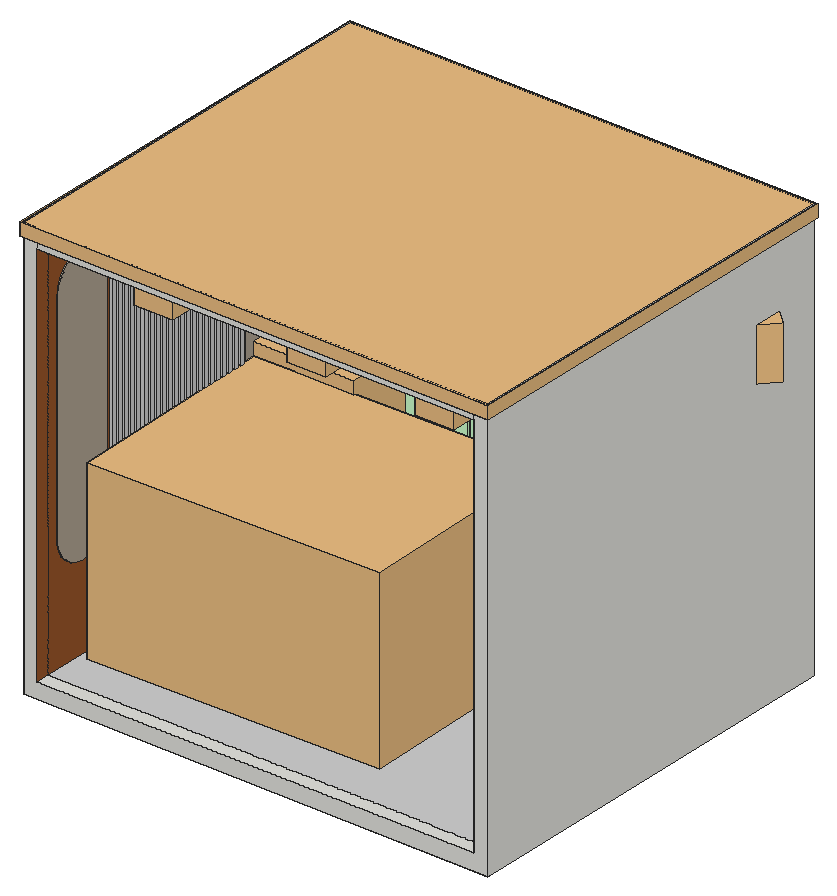
# SketchUp Ruby script. Lengths in inches.
U = 1.inch
M = Sketchup.active_model
def pt(a) = Geom::Point3d.new(a.map { |v| v * U })
def face(e, loops, mat)
  f = e.add_face(loops[0].map { |a| pt(a) })
  loops[1..].each { |l| e.add_face(l.map { |a| pt(a) }).erase! }
  f.material = f.back_material = mat if mat
  f
end
# faces: each face lists its corners as indices into pts; further lists are holes
def faces(e, pts, list, mat = nil) = list.each { |f| face(e, (f[0].is_a?(Array) ? f : [f]).map { |l| l.map { |i| pts[i] } }, mat) }
# xy, xz, yz: faces in a plane at the given z, y or x. An outline is a flat list of corners, or four numbers for a rectangle; further outlines are holes
def ring(l) = l.size == 4 ? [[l[0], l[1]], [l[2], l[1]], [l[2], l[3]], [l[0], l[3]]] : l.each_slice(2).to_a
def flat(e, list, mat, &to3) = list.each { |f| face(e, (f[0].is_a?(Array) ? f : [f]).map { |l| ring(l).map { |u, v| to3.(u, v) } }, mat) }
def xy(e, z, list, mat = nil) = flat(e, list, mat) { |x, y| [x, y, z] }
def xz(e, y, list, mat = nil) = flat(e, list, mat) { |x, z| [x, y, z] }
def yz(e, x, list, mat = nil) = flat(e, list, mat) { |y, z| [x, y, z] }
def lines(e, pts, list) = list.each { |a, b| e.add_line(pt(pts[a]), pt(pts[b])) }
# prism: a flat outline (further loops are holes) pulled along v
def prism(e, loops, v, mat = nil)
  f = face(e, loops, mat); d = Geom::Vector3d.new(v.map { |x| x * U })
  f.pushpull(f.normal.samedirection?(d) ? d.length : -d.length)
end
def box(e, o, s, mat = nil) = prism(e, [[o, [o[0] + s[0], o[1], o[2]], [o[0] + s[0], o[1] + s[1], o[2]], [o[0], o[1] + s[1], o[2]]]], [0, 0, s[2]], mat)
def at(x, y, z, deg = 0) = Geom::Transformation.translation(pt([x, y, z])) * Geom::Transformation.rotation(ORIGIN, Z_AXIS, deg.degrees)
def axes(o, x, y, z) = Geom::Transformation.new([*x, 0, *y, 0, *z, 0, *pt(o).to_a, 1])
def part(name) = M.definitions.add(name)
# library, detail: a bought-in or finely detailed component or shape, given as its bounding box
def library(name, o, s) = part(name).tap { |d| box(d.entities, o, s) }
def detail(e, o, s) = box(e.add_group.entities, o, s)
def put(e, d, t, mat = nil) = e.add_instance(d, t).tap { |i| i.material = mat if mat }
def group(e, t, mat = nil) = e.add_group.tap { |g| g.transformation = t; g.material = mat if mat }.entities
root = M.entities
M.materials.add("[0007_MistyRose]").color = [175, 163, 145]
M.materials.add("[0032_Moccasin]").color = [255, 228, 181]
M.materials.add("[0035_Tan]").color = [210, 180, 140]
M.materials.add("[0067_PaleGreen]").color = [152, 251, 152]
M.materials.add("[Carrera Marble]").color = [207, 207, 207]
M.materials.add("[Color C01]").color = [255, 229, 204]
M.materials.add("[Color G01]").color = [204, 255, 204]
M.materials.add("[Color M04]").color = [142, 142, 142]
M.materials.add("[Mirror 02]").color = [229, 229, 229]
M.materials.add("[Wood Cherry Original]").color = [152, 86, 42]
c1 = library("Spot Light",[-5.1,-5.1,-11.05],[10.2,10.2,11.05])
c2 = library("Spot Light\#1",[-5.1,-5.1,-11.05],[10.2,10.2,11.05])
c3 = library("Spot Light\#2",[-5.1,-5.1,-11.05],[10.2,10.2,11.05])
c4 = library("Spot Light\#3",[-5.1,-5.1,-11.05],[10.2,10.2,11.05])
c5 = library("Spot Light\#4",[-5.1,-5.1,-11.05],[10.2,10.2,11.05])
c6 = library("Spot Light\#5",[-5.1,-5.1,-11.05],[10.2,10.2,11.05])
c7 = library("Spot Light\#7",[-5.1,-5.1,-11.05],[10.2,10.2,11.05])
c8 = library("Tyler Platform Bed",[-34.22,-45.98,0],[68.44,91.98,40.05])
c9 = library("False Aralia 002",[-20.33,-19.19,0],[40.48,38.23,49.87])
c10 = library("Books 297 001 004",[-3.55,-2.96,-0.03],[7.44,5.56,6.72])
c11 = library("Toy 155 013",[-1.73,-1.4375,0],[3.14,2.99,4.15])
c12 = library("Candle 003",[-2.76,-2.76,0],[5.52,5.52,9.79])
c13 = library("Peperomia 450 001",[-6.6875,-10.1875,-9.42],[16.7,12.74,19.03])
c14 = library("Door 243 059",[-21.8,-2.74,0],[43.6,5.48,83.78])
c15 = library("Television screen",[0,1.41,1.14],[35.92,0.28,20.21])
c16 = library("Dome Light",[-12,-12,0],[24,24,12])
c17 = library("Group\#2",[-0.5,-0.5,0],[122.125,107.5,3.25])
c18 = library("Group\#3",[-0.5,-0.5,0],[93.47,84.17,1.0625])
c19 = library("Group\#4",[-0.5,-0.5,0],[1.8125,34.77,40.81])
c20 = library("Group\#5",[-0.5,-0.5,0],[1.8125,35.32,39.97])
c21 = library("Group\#6",[-0.5,-0.5,0],[1.8125,69.04,80.78])
xy(root,0,[[0,0,121.125,106.5]])
xy(root,4.25,[[3.58,0,117.55,3.58]])
xy(root,4.25,[[3.58,3.58,115.3,3.58,115.3,102.92,111.55,102.92,111.55,106.5,74.8,106.5,74.8,102.92,70.3,102.92,70.3,88.61,3.58,88.61]],"[Carrera Marble]")
xy(root,6.57,[[4.27,86.61,46.77,88.61],[46.96,86.92,69.48,88.61]],"[0067_PaleGreen]")
xy(root,8.19,[[48.58,86.92,67.86,87.48]],"[0067_PaleGreen]")
xy(root,13.1875,[[115.3,87.05,120.8,100.98]],"[Color M04]")
xy(root,20.98,[[115.3,87.05,120.8,100.98]],"[Color M04]")
xy(root,21.98,[[115.3,87.05,120.8,100.98]],"[Color M04]")
xy(root,26.6875,[[3.58,47.13,4.8125,48.23],[3.58,49.22,4.8125,50.2],[3.58,51.19,4.8125,52.17],[3.58,53.16,4.8125,54.14],[3.58,55.13,4.8125,56.11],
  [3.58,57.17,4.8125,58.08],[3.58,59.07,4.8125,60.05],[3.58,61.04,4.8125,62.02],[3.58,63.01,4.8125,63.99],[3.58,64.8,4.8125,65.96]])
xy(root,26.6875,[[3.58,23.42,4.52,24.59],[3.58,25.58,4.52,26.56],[3.58,27.55,4.52,28.53],[3.58,29.52,4.52,30.5],[3.58,31.49,4.52,32.47],
  [3.58,33.46,4.8125,34.4375],[3.58,35.43,4.8125,36.41],[3.58,37.4,4.8125,38.38],[3.58,39.37,4.8125,40.35],[3.58,41.28,4.8125,42.32],
  [3.58,43.3125,4.8125,44.29],[3.58,45.28,4.8125,46.26]],"[Carrera Marble]")
xy(root,29.77,[[115.3,87.05,120.8,100.98]],"[Color M04]")
xy(root,30.77,[[115.3,87.05,120.8,100.98]],"[Color M04]")
xy(root,38.5625,[[115.3,87.05,120.8,100.98]],"[Color M04]")
xy(root,39.5625,[[115.3,87.05,120.8,100.98]],"[Color M04]")
xy(root,47.35,[[115.3,87.05,120.8,100.98]],"[Color M04]")
xy(root,48.35,[[115.3,87.05,120.8,100.98]],"[Color M04]")
xy(root,56.15,[[115.3,87.05,120.8,100.98]],"[Color M04]")
xy(root,57.15,[[115.3,87.05,120.8,100.98]],"[Color M04]")
xy(root,64.9375,[[115.3,87.05,120.8,100.98]],"[Color M04]")
xy(root,65.9375,[[115.3,87.05,120.8,100.98]],"[Color M04]")
xy(root,73.73,[[115.3,87.05,120.8,100.98]],"[Color M04]")
xy(root,74.73,[[115.3,87.05,120.8,100.98]],"[Color M04]")
xy(root,82.52,[[115.3,87.05,120.8,100.98]],"[Color M04]")
xy(root,83.52,[[115.3,87.05,120.8,100.98]],"[Color M04]")
xy(root,88.1875,[[74.8,102.92,111.55,106.5]])
xy(root,90.58,[[48.58,86.92,67.86,87.48]],"[0067_PaleGreen]")
xy(root,92.21,[[4.27,86.61,46.77,88.61],[46.96,86.92,69.48,88.61]],"[Color G01]")
xy(root,92.3125,[[116.11,14.57,116.73,82.61]])
xy(root,92.3125,[[115.3,87.05,120.8,100.98]],"[Color M04]")
xy(root,93.21,[[3.58,88.61,70.3,102.92]],"[0032_Moccasin]")
xy(root,99.8125,[[3.58,23.42,4.52,24.59],[3.58,25.58,4.52,26.56],[3.58,27.55,4.52,28.53],[3.58,29.52,4.52,30.5],[3.58,31.49,4.52,32.47],
  [3.58,33.46,4.8125,34.4375],[3.58,35.43,4.8125,36.41],[3.58,37.4,4.8125,38.38],[3.58,39.37,4.8125,40.35],[3.58,41.28,4.8125,42.32],
  [3.58,43.3125,4.8125,44.29],[3.58,45.28,4.8125,46.26],[3.58,47.13,4.8125,48.23],[3.58,49.22,4.8125,50.2],[3.58,51.19,4.8125,52.17],
  [3.58,53.16,4.8125,54.14],[3.58,55.13,4.8125,56.11],[3.58,57.17,4.8125,58.08],[3.58,59.07,4.8125,60.05],[3.58,61.04,4.8125,62.02],
  [3.58,63.01,4.8125,63.99],[3.58,64.8,4.8125,65.96]],"[Carrera Marble]")
xy(root,103.5,[[[18.2,9.625,17.55,9.67,16.91,9.8,16.29,10.01,15.7,10.3,15.16,10.66,14.67,11.09,14.24,11.58,13.875,12.125,13.58,12.71,13.375,13.33,13.25,13.97,13.2,14.625,13.2,88.3,13.25,88.95,13.375,89.59,13.58,90.21,13.875,90.8,14.24,91.34,14.67,91.83,15.16,92.26,15.7,92.625,16.29,92.92,16.91,93.125,17.55,93.25,18.2,93.3,100.67,93.3,101.32,93.25,101.96,93.125,102.58,92.92,103.17,92.625,103.71,92.26,104.21,91.83,104.64,91.34,105,90.8,105.29,90.21,105.5,89.59,105.63,88.95,105.67,88.3,105.67,14.625,105.63,13.97,105.5,13.33,105.29,12.71,105,12.125,104.64,11.58,104.21,11.09,103.71,10.66,103.17,10.3,102.58,10.01,101.96,9.8,101.32,9.67,100.67,9.625],[39.02,30.45,79.85,30.45,80.5,30.49,81.15,30.62,81.76,30.83,82.35,31.12,82.89,31.48,83.39,31.91,83.82,32.4,84.18,32.95,84.47,33.53,84.68,34.15,84.81,34.79,84.85,35.45,84.85,67.48,84.81,68.13,84.68,68.77,84.47,69.39,84.18,69.98,83.82,70.52,83.39,71.01,82.89,71.44,82.35,71.81,81.76,72.1,81.15,72.31,80.5,72.43,79.85,72.48,39.02,72.48,38.37,72.43,37.73,72.31,37.11,72.1,36.52,71.81,35.98,71.44,35.49,71.01,35.06,70.52,34.69,69.98,34.4,69.39,34.19,68.77,34.07,68.13,34.02,67.48,34.02,35.45,34.07,34.79,34.19,34.15,34.4,33.53,34.69,32.95,35.06,32.4,35.49,31.91,35.98,31.48,36.52,31.12,37.11,30.83,37.73,30.62,38.37,30.49],[22.83,78.98,23.7,79.1,24.52,79.44,25.22,79.97,25.75,80.67,26.09,81.48,26.2,82.36,26.09,83.23,25.75,84.05,25.22,84.74,24.52,85.28,23.7,85.62,22.83,85.73,21.96,85.62,21.14,85.28,20.44,84.74,19.91,84.05,19.57,83.23,19.45,82.36,19.57,81.48,19.91,80.67,20.44,79.97,21.14,79.44,21.96,79.1],[96.05,79.11,96.89,79.22,97.67,79.54,98.34,80.06,98.86,80.73,99.18,81.52,99.3,82.36,99.18,83.2,98.86,83.98,98.34,84.66,97.67,85.17,96.89,85.5,96.05,85.61,95.2,85.5,94.42,85.17,93.75,84.66,93.23,83.98,92.91,83.2,92.8,82.36,92.91,81.52,93.23,80.73,93.75,80.06,94.42,79.54,95.2,79.22],[96.05,15.87,96.84,15.97,97.58,16.28,98.21,16.76,98.7,17.4,99,18.14,99.11,18.93,99,19.72,98.7,20.46,98.21,21.1,97.58,21.58,96.84,21.89,96.05,21.99,95.25,21.89,94.51,21.58,93.88,21.1,93.39,20.46,93.09,19.72,92.98,18.93,93.09,18.14,93.39,17.4,93.88,16.76,94.51,16.28,95.25,15.97],[22.83,16.06,23.57,16.15,24.27,16.44,24.86,16.9,25.32,17.49,25.61,18.1875,25.7,18.93,25.61,19.67,25.32,20.37,24.86,20.96,24.27,21.42,23.57,21.71,22.83,21.81,22.09,21.71,21.39,21.42,20.8,20.96,20.34,20.37,20.05,19.67,19.95,18.93,20.05,18.1875,20.34,17.49,20.8,16.9,21.39,16.44,22.09,16.15],[62.49,80,63.1,80.08,63.67,80.3125,64.15,80.6875,64.53,81.18,64.76,81.75,64.85,82.36,64.76,82.97,64.53,83.54,64.15,84.03,63.67,84.4,63.1,84.64,62.49,84.72,61.875,84.64,61.3,84.4,60.82,84.03,60.44,83.54,60.21,82.97,60.125,82.36,60.21,81.75,60.44,81.18,60.82,80.6875,61.3,80.3125,61.875,80.08],[62.49,16.81,63.04,16.88,63.55,17.09,63.99,17.43,64.33,17.87,64.54,18.38,64.61,18.93,64.54,19.48,64.33,19.99,63.99,20.43,63.55,20.77,63.04,20.98,62.49,21.06,61.94,20.98,61.42,20.77,60.98,20.43,60.64,19.99,60.43,19.48,60.36,18.93,60.43,18.38,60.64,17.87,60.98,17.43,61.42,17.09,61.94,16.88]]],"[Color M04]")
xy(root,103.75,[[96.05,79.11,95.2,79.22,94.42,79.54,93.75,80.06,93.23,80.73,92.91,81.52,92.8,82.36,92.91,83.2,93.23,83.98,93.75,84.66,94.42,85.17,95.2,85.5,96.05,85.61,96.89,85.5,97.67,85.17,98.34,84.66,98.86,83.98,99.18,83.2,99.3,82.36,99.18,81.52,98.86,80.73,98.34,80.06,97.67,79.54,96.89,79.22]],"[Color M04]")
xy(root,103.8125,[[22.83,16.06,22.09,16.15,21.39,16.44,20.8,16.9,20.34,17.49,20.05,18.1875,19.95,18.93,20.05,19.67,20.34,20.37,20.8,20.96,21.39,21.42,22.09,21.71,22.83,21.81,23.57,21.71,24.27,21.42,24.86,20.96,25.32,20.37,25.61,19.67,25.7,18.93,25.61,18.1875,25.32,17.49,24.86,16.9,24.27,16.44,23.57,16.15]],"[Color M04]")
xy(root,103.875,[[22.83,78.98,21.96,79.1,21.14,79.44,20.44,79.97,19.91,80.67,19.57,81.48,19.45,82.36,19.57,83.23,19.91,84.05,20.44,84.74,21.14,85.28,21.96,85.62,22.83,85.73,23.7,85.62,24.52,85.28,25.22,84.74,25.75,84.05,26.09,83.23,26.2,82.36,26.09,81.48,25.75,80.67,25.22,79.97,24.52,79.44,23.7,79.1],[62.49,80,61.875,80.08,61.3,80.3125,60.82,80.6875,60.44,81.18,60.21,81.75,60.125,82.36,60.21,82.97,60.44,83.54,60.82,84.03,61.3,84.4,61.875,84.64,62.49,84.72,63.1,84.64,63.67,84.4,64.15,84.03,64.53,83.54,64.76,82.97,64.85,82.36,64.76,81.75,64.53,81.18,64.15,80.6875,63.67,80.3125,63.1,80.08]],"[Color M04]")
xy(root,104.0625,[[96.05,15.87,95.25,15.97,94.51,16.28,93.88,16.76,93.39,17.4,93.09,18.14,92.98,18.93,93.09,19.72,93.39,20.46,93.88,21.1,94.51,21.58,95.25,21.89,96.05,21.99,96.84,21.89,97.58,21.58,98.21,21.1,98.7,20.46,99,19.72,99.11,18.93,99,18.14,98.7,17.4,98.21,16.76,97.58,16.28,96.84,15.97],[62.49,16.81,61.94,16.88,61.42,17.09,60.98,17.43,60.64,17.87,60.43,18.38,60.36,18.93,60.43,19.48,60.64,19.99,60.98,20.43,61.42,20.77,61.94,20.98,62.49,21.06,63.04,20.98,63.55,20.77,63.99,20.43,64.33,19.99,64.54,19.48,64.61,18.93,64.54,18.38,64.33,17.87,63.99,17.43,63.55,17.09,63.04,16.88]],"[Color M04]")
xy(root,105.375,[[[3.58,0,3.58,102.92,115.3,102.92,115.3,3.58,117.55,3.58,117.55,0],[18.2,9.625,100.67,9.625,101.32,9.67,101.96,9.8,102.58,10.01,103.17,10.3,103.71,10.66,104.21,11.09,104.64,11.58,105,12.125,105.29,12.71,105.5,13.33,105.63,13.97,105.67,14.625,105.67,88.3,105.63,88.95,105.5,89.59,105.29,90.21,105,90.8,104.64,91.34,104.21,91.83,103.71,92.26,103.17,92.625,102.58,92.92,101.96,93.125,101.32,93.25,100.67,93.3,18.2,93.3,17.55,93.25,16.91,93.125,16.29,92.92,15.7,92.625,15.16,92.26,14.67,91.83,14.24,91.34,13.875,90.8,13.58,90.21,13.375,89.59,13.25,88.95,13.2,88.3,13.2,14.625,13.25,13.97,13.375,13.33,13.58,12.71,13.875,12.125,14.24,11.58,14.67,11.09,15.16,10.66,15.7,10.3,16.29,10.01,16.91,9.8,17.55,9.67]]],"[Color C01]")
xy(root,109.25,[[39.02,30.45,38.37,30.49,37.73,30.62,37.11,30.83,36.52,31.12,35.98,31.48,35.49,31.91,35.06,32.4,34.69,32.95,34.4,33.53,34.19,34.15,34.07,34.79,34.02,35.45,34.02,67.48,34.07,68.13,34.19,68.77,34.4,69.39,34.69,69.98,35.06,70.52,35.49,71.01,35.98,71.44,36.52,71.81,37.11,72.1,37.73,72.31,38.37,72.43,39.02,72.48,79.85,72.48,80.5,72.43,81.15,72.31,81.76,72.1,82.35,71.81,82.89,71.44,83.39,71.01,83.82,70.52,84.18,69.98,84.47,69.39,84.68,68.77,84.81,68.13,84.85,67.48,84.85,35.45,84.81,34.79,84.68,34.15,84.47,33.53,84.18,32.95,83.82,32.4,83.39,31.91,82.89,31.48,82.35,31.12,81.76,30.83,81.15,30.62,80.5,30.49,79.85,30.45]],"[Color M04]")
xz(root,0,[[0,0,121.125,0,121.125,110.375,117.55,110.375,117.55,4.25,3.58,4.25,3.58,110.375,0,110.375],[3.58,105.375,117.55,110.375]])
xz(root,3.58,[[115.3,4.25,117.55,105.375]],"[Color C01]")
xz(root,9.625,[[18.2,103.5,100.67,104.3125]],"[Color M04]")
xz(root,14.57,[[116.11,11.53,116.73,92.3125]])
xz(root,23.42,[[3.58,26.6875,4.52,99.8125]],"[Carrera Marble]")
xz(root,24.59,[[3.58,26.6875,4.52,99.8125]],"[Carrera Marble]")
xz(root,25.58,[[3.58,26.6875,4.52,99.8125]],"[Carrera Marble]")
xz(root,26.56,[[3.58,26.6875,4.52,99.8125]],"[Carrera Marble]")
xz(root,27.55,[[3.58,26.6875,4.52,99.8125]],"[Carrera Marble]")
xz(root,28.53,[[3.58,26.6875,4.52,99.8125]],"[Carrera Marble]")
xz(root,29.52,[[3.58,26.6875,4.52,99.8125]],"[Carrera Marble]")
xz(root,30.45,[[39.02,103.5,79.85,107.125]],"[Color M04]")
xz(root,30.5,[[3.58,26.6875,4.52,99.8125]],"[Carrera Marble]")
xz(root,31.49,[[3.58,26.6875,4.52,99.8125]],"[Carrera Marble]")
xz(root,32.47,[[3.58,26.6875,4.52,99.8125]],"[Carrera Marble]")
xz(root,33.46,[[3.58,26.6875,4.8125,99.8125]],"[Carrera Marble]")
xz(root,34.4375,[[3.58,26.6875,4.8125,99.8125]],"[Carrera Marble]")
xz(root,35.43,[[3.58,26.6875,4.8125,99.8125]],"[Carrera Marble]")
xz(root,36.41,[[3.58,26.6875,4.8125,99.8125]],"[Carrera Marble]")
xz(root,37.4,[[3.58,26.6875,4.8125,99.8125]],"[Carrera Marble]")
xz(root,38.38,[[3.58,26.6875,4.8125,99.8125]],"[Carrera Marble]")
xz(root,39.37,[[3.58,26.6875,4.8125,99.8125]],"[Carrera Marble]")
xz(root,40.35,[[3.58,26.6875,4.8125,99.8125]],"[Carrera Marble]")
xz(root,41.28,[[3.58,26.6875,4.8125,99.8125]],"[Carrera Marble]")
xz(root,42.32,[[3.58,26.6875,4.8125,99.8125]],"[Carrera Marble]")
xz(root,43.3125,[[3.58,26.6875,4.8125,99.8125]],"[Carrera Marble]")
xz(root,44.29,[[3.58,26.6875,4.8125,99.8125]],"[Carrera Marble]")
xz(root,45.28,[[3.58,26.6875,4.8125,99.8125]],"[Carrera Marble]")
xz(root,46.26,[[3.58,26.6875,4.8125,99.8125]],"[Carrera Marble]")
xz(root,47.13,[[3.58,26.6875,4.8125,99.8125]],"[Carrera Marble]")
xz(root,48.23,[[3.58,26.6875,4.8125,99.8125]],"[Carrera Marble]")
xz(root,49.22,[[3.58,26.6875,4.8125,99.8125]],"[Carrera Marble]")
xz(root,50.2,[[3.58,26.6875,4.8125,99.8125]],"[Carrera Marble]")
xz(root,51.19,[[3.58,26.6875,4.8125,99.8125]],"[Carrera Marble]")
xz(root,52.17,[[3.58,26.6875,4.8125,99.8125]],"[Carrera Marble]")
xz(root,53.16,[[3.58,26.6875,4.8125,99.8125]],"[Carrera Marble]")
xz(root,54.14,[[3.58,26.6875,4.8125,99.8125]],"[Carrera Marble]")
xz(root,55.13,[[3.58,26.6875,4.8125,99.8125]],"[Carrera Marble]")
xz(root,56.11,[[3.58,26.6875,4.8125,99.8125]],"[Carrera Marble]")
xz(root,57.17,[[3.58,26.6875,4.8125,99.8125]],"[Carrera Marble]")
xz(root,58.08,[[3.58,26.6875,4.8125,99.8125]],"[Carrera Marble]")
xz(root,59.07,[[3.58,26.6875,4.8125,99.8125]],"[Carrera Marble]")
xz(root,60.05,[[3.58,26.6875,4.8125,99.8125]],"[Carrera Marble]")
xz(root,61.04,[[3.58,26.6875,4.8125,99.8125]],"[Carrera Marble]")
xz(root,62.02,[[3.58,26.6875,4.8125,99.8125]],"[Carrera Marble]")
xz(root,63.01,[[3.58,26.6875,4.8125,99.8125]],"[Carrera Marble]")
xz(root,63.99,[[3.58,26.6875,4.8125,99.8125]],"[Carrera Marble]")
xz(root,64.8,[[3.58,26.6875,4.8125,99.8125]],"[Carrera Marble]")
xz(root,65.96,[[3.58,26.6875,4.8125,99.8125]],"[Carrera Marble]")
xz(root,72.48,[[39.02,103.5,79.85,107.125]],"[Color M04]")
xz(root,86.61,[[4.27,6.57,46.77,92.21]],"[Color G01]")
xz(root,86.61,[[58.22,21.78,60.06,22.05,61.74,22.83,63.13,24.0625,64.12,25.64,64.57,27.29,64.57,77.72,64.36,79.37,63.72,80.9,62.71,82.22,61.4,83.23,59.86,83.86,58.22,84.08,56.57,83.86,55.04,83.23,53.73,82.22,52.72,80.9,52.08,79.37,51.86,77.72,51.86,27.29,52.32,25.64,53.3,24.0625,54.7,22.83,56.38,22.05]],"[Mirror 02]")
xz(root,86.92,[[[46.96,6.57,69.48,92.21],[48.58,8.19,67.86,90.58]]],"[Color G01]")
xz(root,87.05,[[115.3,20.98,120.8,21.98],[115.3,29.77,120.8,30.77],[115.3,38.5625,120.8,39.5625],[115.3,47.35,120.8,48.35],[115.3,56.15,120.8,57.15],
  [115.3,64.9375,120.8,65.9375],[115.3,73.73,120.8,74.73],[115.3,82.52,120.8,83.52]])
xz(root,87.05,[[115.3,13.1875,120.8,20.98],[115.3,21.98,120.8,29.77],[115.3,30.77,120.8,38.5625],[115.3,39.5625,120.8,47.35],[115.3,48.35,120.8,56.15],
  [115.3,57.15,120.8,64.9375],[115.3,65.9375,120.8,73.73],[115.3,74.73,120.8,82.52],[115.3,83.52,120.8,92.3125]],"[Color M04]")
xz(root,87.48,[[[48.58,8.19,67.86,90.58],[58.22,21.78,56.38,22.05,54.7,22.83,53.3,24.0625,52.32,25.64,51.86,27.29,51.83,27.43,51.86,29.28,51.86,77.72,52.08,79.37,52.72,80.9,53.73,82.22,55.04,83.23,56.57,83.86,58.22,84.08,59.86,83.86,61.4,83.23,62.71,82.22,63.72,80.9,64.36,79.37,64.57,77.72,64.57,29.28,64.61,27.43,64.57,27.29,64.12,25.64,63.13,24.0625,61.74,22.83,60.06,22.05]],[51.86,27.29,51.86,29.28,51.83,27.43],[64.57,27.29,64.61,27.43,64.57,29.28]],"[Color G01]")
xz(root,88.61,[[46.77,6.57,46.96,90.89]])
xz(root,88.61,[[[3.58,4.25,70.3,93.21],[4.27,6.57,4.27,92.21,46.77,92.21,46.77,90.89,46.96,90.89,46.96,92.21,69.48,92.21,69.48,6.57]]],"[0032_Moccasin]")
xz(root,93.3,[[18.2,103.5,100.67,104.3125],[18.2,104.3125,100.67,105.375]],"[Color M04]")
xz(root,100.98,[[115.3,13.1875,120.8,20.98],[115.3,21.98,120.8,29.77],[115.3,30.77,120.8,38.5625],[115.3,39.5625,120.8,47.35],[115.3,48.35,120.8,56.15],
  [115.3,57.15,120.8,64.9375],[115.3,65.9375,120.8,73.73],[115.3,74.73,120.8,82.52],[115.3,83.52,120.8,92.3125]],"[Color M04]")
xz(root,102.92,[[70.3,4.25,74.8,4.25,74.8,88.1875,111.55,88.1875,111.55,4.25,115.3,4.25,115.3,105.375,3.58,105.375,3.58,93.21,70.3,93.21]],"[Color C01]")
xz(root,106.5,[[[0,0,121.125,110.375],[74.8,4.25,111.55,88.1875]]])
yz(root,0,[[0,0,106.5,110.375]])
yz(root,3.58,[[0,4.25,3.58,105.375],[[3.58,4.25,88.61,4.25,88.61,93.21,102.92,93.21,102.92,105.375,3.58,105.375],[64.8,26.6875,65.96,99.8125],[23.42,26.6875,24.59,99.8125],[47.13,26.6875,48.23,99.8125],[41.28,26.6875,42.32,99.8125],[61.04,26.6875,62.02,99.8125],[53.16,26.6875,54.14,99.8125],[49.22,26.6875,50.2,99.8125],[45.28,26.6875,46.26,99.8125],[37.4,26.6875,38.38,99.8125],[33.46,26.6875,34.4375,99.8125],[29.52,26.6875,30.5,99.8125],[27.55,26.6875,28.53,99.8125],[25.58,26.6875,26.56,99.8125],[63.01,26.6875,63.99,99.8125],[59.07,26.6875,60.05,99.8125],[55.13,26.6875,56.11,99.8125],[51.19,26.6875,52.17,99.8125],[43.3125,26.6875,44.29,99.8125],[39.37,26.6875,40.35,99.8125],[35.43,26.6875,36.41,99.8125],[31.49,26.6875,32.47,99.8125],[57.17,26.6875,58.08,99.8125]]],"[Wood Cherry Original]")
yz(root,4.27,[[86.61,6.57,88.61,92.21]],"[0067_PaleGreen]")
yz(root,4.52,[[23.42,26.6875,24.59,99.8125],[25.58,26.6875,26.56,99.8125],[27.55,26.6875,28.53,99.8125],[29.52,26.6875,30.5,99.8125],[31.49,26.6875,32.47,99.8125]],"[Carrera Marble]")
yz(root,4.8125,[[33.46,26.6875,34.4375,99.8125],[35.43,26.6875,36.41,99.8125],[37.4,26.6875,38.38,99.8125],[39.37,26.6875,40.35,99.8125],[41.28,26.6875,42.32,99.8125],
  [43.3125,26.6875,44.29,99.8125],[45.28,26.6875,46.26,99.8125],[47.13,26.6875,48.23,99.8125],[49.22,26.6875,50.2,99.8125],[51.19,26.6875,52.17,99.8125],
  [53.16,26.6875,54.14,99.8125],[55.13,26.6875,56.11,99.8125],[57.17,26.6875,58.08,99.8125],[59.07,26.6875,60.05,99.8125],[61.04,26.6875,62.02,99.8125],
  [63.01,26.6875,63.99,99.8125],[64.8,26.6875,65.96,99.8125]],"[Carrera Marble]")
yz(root,13.2,[[14.625,103.5,88.3,104.3125]],"[Color M04]")
yz(root,34.02,[[35.45,103.5,67.48,107.125]],"[Color M04]")
yz(root,46.77,[[86.61,6.57,88.61,92.21]],"[Color G01]")
yz(root,46.96,[[86.92,6.57,88.61,92.21]],"[Color G01]")
yz(root,48.58,[[86.92,8.19,87.48,90.58]],"[Color G01]")
yz(root,51.86,[[86.61,27.29,87.48,29.28],[86.61,29.28,87.48,77.72]],"[Mirror 02]")
yz(root,64.57,[[86.61,27.29,87.48,29.28],[86.61,29.28,87.48,77.72]],"[Mirror 02]")
yz(root,67.86,[[86.92,8.19,87.48,90.58]],"[Color G01]")
yz(root,69.48,[[86.92,6.57,88.61,92.21]],"[Color G01]")
yz(root,70.3,[[88.61,4.25,102.92,93.21]],"[0032_Moccasin]")
yz(root,74.8,[[102.92,4.25,106.5,88.1875]])
yz(root,84.85,[[35.45,103.5,67.48,107.125]],"[Color M04]")
yz(root,105.67,[[14.625,103.5,88.3,104.3125]],"[Color M04]")
yz(root,111.55,[[102.92,4.25,106.5,88.1875]])
yz(root,115.3,[[14.57,11.53,19.38,12.25,24.05,13.59,28.52,15.51,32.69,18,36.51,21.01,39.91,24.49,42.83,28.375,45.23,32.61,47.05,37.11,48.28,41.82,48.89,46.64,48.87,51.5,48.84,56.37,49.43,61.2,50.62,65.91,52.4,70.4375,54.74,74.71,57.59,78.64,60.92,82.1875,64.68,85.28,68.79,87.88,73.19,89.94,77.83,91.42,82.61,92.3125,82.61,11.53]],"[0035_Tan]")
yz(root,115.3,[[[3.58,4.25,102.92,105.375],[14.57,11.53,82.61,92.3125],[87.05,13.1875,100.98,13.1875,100.98,92.3125,87.05,92.3125,87.05,83.52,100.98,83.52,100.98,82.52,87.05,82.52,87.05,74.73,100.98,74.73,100.98,73.73,87.05,73.73,87.05,65.9375,100.98,65.9375,100.98,64.9375,87.05,64.9375,87.05,57.15,100.98,57.15,100.98,56.15,87.05,56.15,87.05,48.35,100.98,48.35,100.98,47.35,87.05,47.35,87.05,39.5625,100.98,39.5625,100.98,38.5625,87.05,38.5625,87.05,30.77,100.98,30.77,100.98,29.77,87.05,29.77,87.05,21.98,100.98,21.98,100.98,20.98,87.05,20.98]]],"[Color C01]")
yz(root,116.73,[[14.57,11.53,14.57,92.3125,82.61,92.3125,77.83,91.42,73.19,89.94,68.79,87.88,64.68,85.28,60.92,82.1875,57.59,78.64,54.74,74.71,52.4,70.4375,50.62,65.91,49.43,61.2,48.84,56.37,48.87,51.5,48.89,46.64,48.28,41.82,47.05,37.11,45.23,32.61,42.83,28.375,39.91,24.49,36.51,21.01,32.69,18,28.52,15.51,24.05,13.59,19.38,12.25]],"[0035_Tan]")
yz(root,117.55,[[0,4.25,3.58,105.375]])
yz(root,120.8,[[87.05,13.1875,100.98,20.98],[87.05,21.98,100.98,29.77],[87.05,30.77,100.98,38.5625],[87.05,39.5625,100.98,47.35],[87.05,48.35,100.98,56.15],
  [87.05,57.15,100.98,64.9375],[87.05,65.9375,100.98,73.73],[87.05,74.73,100.98,82.52],[87.05,83.52,100.98,92.3125]],"[Color M04]")
yz(root,121.125,[[0,0,106.5,110.375]])
p = [[116.73,19.38,12.25],[116.11,19.38,12.25],[116.11,14.57,11.53],[116.73,14.57,11.53],[116.73,24.05,13.59],[116.11,24.05,13.59],
  [116.73,28.52,15.51],[116.11,28.52,15.51],[116.73,32.69,18],[116.11,32.69,18],[116.73,36.51,21.01],[116.11,36.51,21.01],
  [116.73,39.91,24.49],[116.11,39.91,24.49],[56.38,87.48,22.05],[58.22,87.48,21.78],[58.22,86.61,21.78],[56.38,86.61,22.05],
  [60.06,87.48,22.05],[60.06,86.61,22.05],[54.7,87.48,22.83],[54.7,86.61,22.83],[61.74,87.48,22.83],[61.74,86.61,22.83],
  [53.3,87.48,24.0625],[53.3,86.61,24.0625],[63.13,87.48,24.0625],[63.13,86.61,24.0625],[52.32,87.48,25.64],[52.32,86.61,25.64],
  [64.12,87.48,25.64],[64.12,86.61,25.64],[116.73,42.83,28.375],[116.11,42.83,28.375],[51.86,87.48,27.29],[51.86,86.61,27.29],
  [64.57,87.48,27.29],[64.57,86.61,27.29],[116.73,45.23,32.61],[116.11,45.23,32.61],[116.73,47.05,37.11],[116.11,47.05,37.11],
  [116.73,48.28,41.82],[116.11,48.28,41.82],[116.73,48.89,46.64],[116.11,48.89,46.64],[116.73,48.87,51.5],[116.11,48.87,51.5],
  [116.73,48.84,56.37],[116.11,48.84,56.37],[116.73,49.43,61.2],[116.11,49.43,61.2],[116.73,50.62,65.91],[116.11,50.62,65.91],
  [116.73,52.4,70.4375],[116.11,52.4,70.4375],[116.73,54.74,74.71],[116.11,54.74,74.71],[116.73,57.59,78.64],[116.11,57.59,78.64],
  [52.08,87.48,79.37],[51.86,87.48,77.72],[51.86,86.61,77.72],[52.08,86.61,79.37],[64.57,87.48,77.72],[64.36,87.48,79.37],
  [64.36,86.61,79.37],[64.57,86.61,77.72],[116.73,60.92,82.1875],[116.11,60.92,82.1875],[52.72,87.48,80.9],[52.72,86.61,80.9],
  [63.72,87.48,80.9],[63.72,86.61,80.9],[53.73,87.48,82.22],[53.73,86.61,82.22],[62.71,87.48,82.22],[62.71,86.61,82.22],
  [116.73,64.68,85.28],[116.11,64.68,85.28],[55.04,87.48,83.23],[55.04,86.61,83.23],[61.4,87.48,83.23],[61.4,86.61,83.23],
  [56.57,87.48,83.86],[56.57,86.61,83.86],[59.86,87.48,83.86],[59.86,86.61,83.86],[58.22,87.48,84.08],[58.22,86.61,84.08],
  [116.73,68.79,87.88],[116.11,68.79,87.88],[116.73,73.19,89.94],[116.11,73.19,89.94],[116.73,77.83,91.42],[116.11,77.83,91.42],
  [116.73,82.61,92.3125],[116.11,82.61,92.3125],[18.2,9.625,103.5],[18.2,9.625,104.3125],[17.55,9.67,104.3125],[17.55,9.67,103.5],
  [101.32,9.67,103.5],[101.32,9.67,104.3125],[100.67,9.625,104.3125],[100.67,9.625,103.5],[16.91,9.8,104.3125],[16.91,9.8,103.5],
  [101.96,9.8,103.5],[101.96,9.8,104.3125],[16.29,10.01,104.3125],[16.29,10.01,103.5],[102.58,10.01,103.5],[102.58,10.01,104.3125],
  [15.7,10.3,104.3125],[15.7,10.3,103.5],[103.17,10.3,103.5],[103.17,10.3,104.3125],[15.16,10.66,104.3125],[15.16,10.66,103.5],
  [103.71,10.66,103.5],[103.71,10.66,104.3125],[14.67,11.09,104.3125],[14.67,11.09,103.5],[104.21,11.09,103.5],[104.21,11.09,104.3125],
  [14.24,11.58,104.3125],[14.24,11.58,103.5],[104.64,11.58,103.5],[104.64,11.58,104.3125],[13.875,12.125,104.3125],[13.875,12.125,103.5],
  [105,12.125,103.5],[105,12.125,104.3125],[13.58,12.71,104.3125],[13.58,12.71,103.5],[105.29,12.71,103.5],[105.29,12.71,104.3125],
  [13.375,13.33,104.3125],[13.375,13.33,103.5],[105.5,13.33,103.5],[105.5,13.33,104.3125],[13.25,13.97,104.3125],[13.25,13.97,103.5],
  [105.63,13.97,103.5],[105.63,13.97,104.3125],[13.2,14.625,104.3125],[13.2,14.625,103.5],[105.67,14.625,103.5],[105.67,14.625,104.3125],
  [96.05,15.87,103.5],[95.25,15.97,103.5],[95.25,15.97,104.0625],[96.05,15.87,104.0625],[96.84,15.97,103.5],[96.84,15.97,104.0625],
  [94.51,16.28,103.5],[94.51,16.28,104.0625],[97.58,16.28,103.5],[97.58,16.28,104.0625],[22.83,16.06,103.5],[22.09,16.15,103.5],
  [22.09,16.15,103.8125],[22.83,16.06,103.8125],[23.57,16.15,103.5],[23.57,16.15,103.8125],[21.39,16.44,103.5],[21.39,16.44,103.8125],
  [24.27,16.44,103.5],[24.27,16.44,103.8125],[93.88,16.76,103.5],[93.88,16.76,104.0625],[98.21,16.76,103.5],[98.21,16.76,104.0625],
  [20.8,16.9,103.5],[20.8,16.9,103.8125],[24.86,16.9,103.5],[24.86,16.9,103.8125],[62.49,16.81,103.5],[61.94,16.88,103.5],
  [61.94,16.88,104.0625],[62.49,16.81,104.0625],[63.04,16.88,103.5],[63.04,16.88,104.0625],[93.39,17.4,103.5],[93.39,17.4,104.0625],
  [98.7,17.4,103.5],[98.7,17.4,104.0625],[20.34,17.49,103.5],[20.34,17.49,103.8125],[25.32,17.49,103.5],[25.32,17.49,103.8125],
  [61.42,17.09,103.5],[61.42,17.09,104.0625],[63.55,17.09,103.5],[63.55,17.09,104.0625],[60.98,17.43,103.5],[60.98,17.43,104.0625],
  [63.99,17.43,103.5],[63.99,17.43,104.0625],[60.64,17.87,103.5],[60.64,17.87,104.0625],[64.33,17.87,103.5],[64.33,17.87,104.0625],
  [93.09,18.14,103.5],[93.09,18.14,104.0625],[99,18.14,103.5],[99,18.14,104.0625],[20.05,18.1875,103.5],[20.05,18.1875,103.8125],
  [25.61,18.1875,103.5],[25.61,18.1875,103.8125],[60.43,18.38,103.5],[60.43,18.38,104.0625],[64.54,18.38,103.5],[64.54,18.38,104.0625],
  [92.98,18.93,103.5],[92.98,18.93,104.0625],[99.11,18.93,103.5],[99.11,18.93,104.0625],[19.95,18.93,103.5],[19.95,18.93,103.8125],
  [25.7,18.93,103.5],[25.7,18.93,103.8125],[60.36,18.93,103.5],[60.36,18.93,104.0625],[64.61,18.93,103.5],[64.61,18.93,104.0625],
  [20.05,19.67,103.5],[20.05,19.67,103.8125],[25.61,19.67,103.5],[25.61,19.67,103.8125],[60.43,19.48,103.5],[60.43,19.48,104.0625],
  [64.54,19.48,103.5],[64.54,19.48,104.0625],[93.09,19.72,103.5],[93.09,19.72,104.0625],[99,19.72,103.5],[99,19.72,104.0625],
  [60.64,19.99,103.5],[60.64,19.99,104.0625],[64.33,19.99,103.5],[64.33,19.99,104.0625],[20.34,20.37,103.5],[20.34,20.37,103.8125],
  [25.32,20.37,103.5],[25.32,20.37,103.8125],[93.39,20.46,103.5],[93.39,20.46,104.0625],[98.7,20.46,103.5],[98.7,20.46,104.0625],
  [60.98,20.43,103.5],[60.98,20.43,104.0625],[63.99,20.43,103.5],[63.99,20.43,104.0625],[20.8,20.96,103.5],[20.8,20.96,103.8125],
  [24.86,20.96,103.5],[24.86,20.96,103.8125],[61.42,20.77,103.5],[61.42,20.77,104.0625],[63.55,20.77,103.5],[63.55,20.77,104.0625],
  [93.88,21.1,103.5],[93.88,21.1,104.0625],[98.21,21.1,103.5],[98.21,21.1,104.0625],[61.94,20.98,103.5],[61.94,20.98,104.0625],
  [63.04,20.98,103.5],[63.04,20.98,104.0625],[21.39,21.42,103.5],[21.39,21.42,103.8125],[24.27,21.42,103.5],[24.27,21.42,103.8125],
  [62.49,21.06,103.5],[62.49,21.06,104.0625],[94.51,21.58,103.5],[94.51,21.58,104.0625],[97.58,21.58,103.5],[97.58,21.58,104.0625],
  [22.09,21.71,103.5],[22.09,21.71,103.8125],[23.57,21.71,103.5],[23.57,21.71,103.8125],[95.25,21.89,103.5],[95.25,21.89,104.0625],
  [96.84,21.89,103.5],[96.84,21.89,104.0625],[22.83,21.81,103.5],[22.83,21.81,103.8125],[96.05,21.99,103.5],[96.05,21.99,104.0625],
  [38.37,30.49,103.5],[38.37,30.49,107.125],[39.02,30.45,107.125],[39.02,30.45,103.5],[79.85,30.45,103.5],[79.85,30.45,107.125],
  [80.5,30.49,107.125],[80.5,30.49,103.5],[37.73,30.62,103.5],[37.73,30.62,107.125],[81.15,30.62,107.125],[81.15,30.62,103.5],
  [37.11,30.83,103.5],[37.11,30.83,107.125],[81.76,30.83,107.125],[81.76,30.83,103.5],[36.52,31.12,103.5],[36.52,31.12,107.125],
  [82.35,31.12,107.125],[82.35,31.12,103.5],[35.98,31.48,103.5],[35.98,31.48,107.125],[82.89,31.48,107.125],[82.89,31.48,103.5],
  [35.49,31.91,103.5],[35.49,31.91,107.125],[83.39,31.91,107.125],[83.39,31.91,103.5],[35.06,32.4,103.5],[35.06,32.4,107.125],
  [83.82,32.4,107.125],[83.82,32.4,103.5],[34.69,32.95,103.5],[34.69,32.95,107.125],[84.18,32.95,107.125],[84.18,32.95,103.5],
  [34.4,33.53,103.5],[34.4,33.53,107.125],[84.47,33.53,107.125],[84.47,33.53,103.5],[34.19,34.15,103.5],[34.19,34.15,107.125],
  [84.68,34.15,107.125],[84.68,34.15,103.5],[34.07,34.79,103.5],[34.07,34.79,107.125],[84.81,34.79,107.125],[84.81,34.79,103.5],
  [34.02,35.45,103.5],[34.02,35.45,107.125],[84.85,35.45,107.125],[84.85,35.45,103.5],[34.07,68.13,103.5],[34.07,68.13,107.125],
  [34.02,67.48,107.125],[34.02,67.48,103.5],[84.85,67.48,103.5],[84.85,67.48,107.125],[84.81,68.13,107.125],[84.81,68.13,103.5],
  [34.19,68.77,103.5],[34.19,68.77,107.125],[84.68,68.77,107.125],[84.68,68.77,103.5],[34.4,69.39,103.5],[34.4,69.39,107.125],
  [84.47,69.39,107.125],[84.47,69.39,103.5],[34.69,69.98,103.5],[34.69,69.98,107.125],[84.18,69.98,107.125],[84.18,69.98,103.5],
  [35.06,70.52,103.5],[35.06,70.52,107.125],[83.82,70.52,107.125],[83.82,70.52,103.5],[35.49,71.01,103.5],[35.49,71.01,107.125],
  [83.39,71.01,107.125],[83.39,71.01,103.5],[35.98,71.44,103.5],[35.98,71.44,107.125],[82.89,71.44,107.125],[82.89,71.44,103.5],
  [36.52,71.81,103.5],[36.52,71.81,107.125],[82.35,71.81,107.125],[82.35,71.81,103.5],[37.11,72.1,103.5],[37.11,72.1,107.125],
  [81.76,72.1,107.125],[81.76,72.1,103.5],[37.73,72.31,103.5],[37.73,72.31,107.125],[81.15,72.31,107.125],[81.15,72.31,103.5],
  [38.37,72.43,103.5],[38.37,72.43,107.125],[80.5,72.43,107.125],[80.5,72.43,103.5],[39.02,72.48,103.5],[39.02,72.48,107.125],
  [79.85,72.48,107.125],[79.85,72.48,103.5],[22.83,78.98,103.5],[21.96,79.1,103.5],[21.96,79.1,103.875],[22.83,78.98,103.875],
  [23.7,79.1,103.5],[23.7,79.1,103.875],[21.14,79.44,103.5],[21.14,79.44,103.875],[24.52,79.44,103.5],[24.52,79.44,103.875],
  [96.05,79.11,103.5],[95.2,79.22,103.5],[95.2,79.22,103.75],[96.05,79.11,103.75],[96.89,79.22,103.5],[96.89,79.22,103.75],
  [94.42,79.54,103.5],[94.42,79.54,103.75],[97.67,79.54,103.5],[97.67,79.54,103.75],[20.44,79.97,103.5],[20.44,79.97,103.875],
  [25.22,79.97,103.5],[25.22,79.97,103.875],[93.75,80.06,103.5],[93.75,80.06,103.75],[98.34,80.06,103.5],[98.34,80.06,103.75],
  [19.91,80.67,103.5],[19.91,80.67,103.875],[25.75,80.67,103.5],[25.75,80.67,103.875],[62.49,80,103.5],[61.875,80.08,103.5],
  [61.875,80.08,103.875],[62.49,80,103.875],[63.1,80.08,103.5],[63.1,80.08,103.875],[61.3,80.3125,103.5],[61.3,80.3125,103.875],
  [63.67,80.3125,103.5],[63.67,80.3125,103.875],[93.23,80.73,103.5],[93.23,80.73,103.75],[98.86,80.73,103.5],[98.86,80.73,103.75],
  [60.82,80.6875,103.5],[60.82,80.6875,103.875],[64.15,80.6875,103.5],[64.15,80.6875,103.875],[19.57,81.48,103.5],[19.57,81.48,103.875],
  [26.09,81.48,103.5],[26.09,81.48,103.875],[60.44,81.18,103.5],[60.44,81.18,103.875],[64.53,81.18,103.5],[64.53,81.18,103.875],
  [92.91,81.52,103.5],[92.91,81.52,103.75],[99.18,81.52,103.5],[99.18,81.52,103.75],[60.21,81.75,103.5],[60.21,81.75,103.875],
  [64.76,81.75,103.5],[64.76,81.75,103.875],[19.45,82.36,103.5],[19.45,82.36,103.875],[26.2,82.36,103.5],[26.2,82.36,103.875],
  [92.8,82.36,103.5],[92.8,82.36,103.75],[99.3,82.36,103.5],[99.3,82.36,103.75],[60.125,82.36,103.5],[60.125,82.36,103.875],
  [64.85,82.36,103.5],[64.85,82.36,103.875],[19.57,83.23,103.5],[19.57,83.23,103.875],[26.09,83.23,103.5],[26.09,83.23,103.875],
  [60.21,82.97,103.5],[60.21,82.97,103.875],[64.76,82.97,103.5],[64.76,82.97,103.875],[92.91,83.2,103.5],[92.91,83.2,103.75],
  [99.18,83.2,103.5],[99.18,83.2,103.75],[60.44,83.54,103.5],[60.44,83.54,103.875],[64.53,83.54,103.5],[64.53,83.54,103.875],
  [19.91,84.05,103.5],[19.91,84.05,103.875],[25.75,84.05,103.5],[25.75,84.05,103.875],[93.23,83.98,103.5],[93.23,83.98,103.75],
  [98.86,83.98,103.5],[98.86,83.98,103.75],[60.82,84.03,103.5],[60.82,84.03,103.875],[64.15,84.03,103.5],[64.15,84.03,103.875],
  [20.44,84.74,103.5],[20.44,84.74,103.875],[25.22,84.74,103.5],[25.22,84.74,103.875],[61.3,84.4,103.5],[61.3,84.4,103.875],
  [63.67,84.4,103.5],[63.67,84.4,103.875],[93.75,84.66,103.5],[93.75,84.66,103.75],[98.34,84.66,103.5],[98.34,84.66,103.75],
  [61.875,84.64,103.5],[61.875,84.64,103.875],[63.1,84.64,103.5],[63.1,84.64,103.875],[62.49,84.72,103.5],[62.49,84.72,103.875],
  [21.14,85.28,103.5],[21.14,85.28,103.875],[24.52,85.28,103.5],[24.52,85.28,103.875],[94.42,85.17,103.5],[94.42,85.17,103.75],
  [97.67,85.17,103.5],[97.67,85.17,103.75],[95.2,85.5,103.5],[95.2,85.5,103.75],[96.89,85.5,103.5],[96.89,85.5,103.75],
  [21.96,85.62,103.5],[21.96,85.62,103.875],[23.7,85.62,103.5],[23.7,85.62,103.875],[96.05,85.61,103.5],[96.05,85.61,103.75],
  [22.83,85.73,103.5],[22.83,85.73,103.875],[13.2,88.3,105.375],[13.25,88.95,105.375],[13.25,88.95,103.5],[13.2,88.3,103.5],
  [13.2,88.3,104.3125],[105.63,88.95,103.5],[105.63,88.95,104.3125],[105.67,88.3,104.3125],[105.67,88.3,103.5],[13.375,89.59,105.375],
  [13.375,89.59,103.5],[105.5,89.59,103.5],[105.5,89.59,104.3125],[13.58,90.21,105.375],[13.58,90.21,103.5],[105.29,90.21,103.5],
  [105.29,90.21,104.3125],[13.875,90.8,105.375],[13.875,90.8,103.5],[105,90.8,103.5],[105,90.8,104.3125],[14.24,91.34,105.375],
  [14.24,91.34,103.5],[104.64,91.34,103.5],[104.64,91.34,104.3125],[14.67,91.83,105.375],[14.67,91.83,103.5],[104.21,91.83,103.5],
  [104.21,91.83,104.3125],[15.16,92.26,105.375],[15.16,92.26,103.5],[103.71,92.26,103.5],[103.71,92.26,104.3125],[15.7,92.625,105.375],
  [15.7,92.625,103.5],[103.17,92.625,103.5],[103.17,92.625,104.3125],[16.29,92.92,105.375],[16.29,92.92,103.5],[102.58,92.92,103.5],
  [102.58,92.92,104.3125],[16.91,93.125,105.375],[16.91,93.125,103.5],[101.96,93.125,103.5],[101.96,93.125,104.3125],[17.55,93.25,105.375],
  [17.55,93.25,103.5],[101.32,93.25,103.5],[101.32,93.25,104.3125],[18.2,93.3,105.375],[18.2,93.3,104.3125],[18.2,93.3,103.5],
  [100.67,93.3,103.5],[100.67,93.3,104.3125],[105.67,88.3,105.375],[105.63,88.95,105.375],[105.5,89.59,105.375],[105.29,90.21,105.375],
  [105,90.8,105.375],[104.64,91.34,105.375],[104.21,91.83,105.375],[103.71,92.26,105.375],[103.17,92.625,105.375],[102.58,92.92,105.375],
  [101.96,93.125,105.375],[101.32,93.25,105.375],[100.67,93.3,105.375],[3.58,3.58,105.375],[3.58,3.58,110.375],[116.125,14.57,94.0625],
  [116.125,14.57,92.3125]]
faces(root,p,[[0,1,2,3],[4,5,1,0],[6,7,5,4],[8,9,7,6],[10,11,9,8],[12,13,11,10],[32,33,13,12],[38,39,33,32],
  [40,41,39,38],[42,43,41,40],[44,45,43,42],[46,47,45,44],[542,543,544,545,546],[543,551,552,544],[551,555,556,552],[555,559,560,556],
  [559,563,564,560],[563,567,568,564],[567,571,572,568],[571,575,576,572],[575,579,580,576],[579,583,584,580],[583,587,588,584],[587,591,592,593,588]])
faces(root,p,[[14,15,16,17],[15,18,19,16],[20,14,17,21],[18,22,23,19],[24,20,21,25],[22,26,27,23],[28,24,25,29],[26,30,31,27],
  [34,28,29,35],[30,36,37,31],[60,61,62,63],[64,65,66,67],[70,60,63,71],[65,72,73,66],[74,70,71,75],[72,76,77,73],
  [80,74,75,81],[76,82,83,77],[84,80,81,85],[82,86,87,83],[88,84,85,89],[86,88,89,87]],"[Mirror 02]")
faces(root,p,[[48,49,47,46],[50,51,49,48],[52,53,51,50],[54,55,53,52],[56,57,55,54],[58,59,57,56],[68,69,59,58],[78,79,69,68],
  [90,91,79,78],[92,93,91,90],[94,95,93,92],[96,97,95,94]],"[Color C01]")
faces(root,p,[[98,99,100,101],[102,103,104,105],[101,100,106,107],[108,109,103,102],[107,106,110,111],[112,113,109,108],[111,110,114,115],[116,117,113,112],
  [115,114,118,119],[120,121,117,116],[119,118,122,123],[124,125,121,120],[123,122,126,127],[128,129,125,124],[127,126,130,131],[132,133,129,128],
  [131,130,134,135],[136,137,133,132],[135,134,138,139],[140,141,137,136],[139,138,142,143],[144,145,141,140],[143,142,146,147],[148,149,145,144],
  [150,151,152,153],[154,150,153,155],[151,156,157,152],[158,154,155,159],[160,161,162,163],[164,160,163,165],[161,166,167,162],[168,164,165,169],
  [156,170,171,157],[172,158,159,173],[166,174,175,167],[176,168,169,177],[178,179,180,181],[182,178,181,183],[170,184,185,171],[186,172,173,187],
  [174,188,189,175],[190,176,177,191],[179,192,193,180],[194,182,183,195],[192,196,197,193],[198,194,195,199],[196,200,201,197],[202,198,199,203],
  [184,204,205,185],[206,186,187,207],[188,208,209,189],[210,190,191,211],[200,212,213,201],[214,202,203,215],[204,216,217,205],[218,206,207,219],
  [208,220,221,209],[222,210,211,223],[212,224,225,213],[226,214,215,227],[220,228,229,221],[230,222,223,231],[224,232,233,225],[234,226,227,235],
  [216,236,237,217],[238,218,219,239],[232,240,241,233],[242,234,235,243],[228,244,245,229],[246,230,231,247],[236,248,249,237],[250,238,239,251],
  [240,252,253,241],[254,242,243,255],[244,256,257,245],[258,246,247,259],[252,260,261,253],[262,254,255,263],[248,264,265,249],[266,250,251,267],
  [260,268,269,261],[270,262,263,271],[256,272,273,257],[274,258,259,275],[268,276,277,269],[276,270,271,277],[264,278,279,265],[280,266,267,281],
  [272,282,283,273],[284,274,275,285],[278,286,287,279],[288,280,281,289],[282,290,291,283],[290,284,285,291],[286,292,293,287],[292,288,289,293],
  [294,295,296,297],[298,299,300,301],[302,303,295,294],[301,300,304,305],[306,307,303,302],[305,304,308,309],[310,311,307,306],[309,308,312,313],
  [314,315,311,310],[313,312,316,317],[318,319,315,314],[317,316,320,321],[322,323,319,318],[321,320,324,325],[326,327,323,322],[325,324,328,329],
  [330,331,327,326],[329,328,332,333],[334,335,331,330],[333,332,336,337],[338,339,335,334],[337,336,340,341],[342,343,339,338],[341,340,344,345],
  [346,347,348,349],[350,351,352,353],[354,355,347,346],[353,352,356,357],[358,359,355,354],[357,356,360,361],[362,363,359,358],[361,360,364,365],
  [366,367,363,362],[365,364,368,369],[370,371,367,366],[369,368,372,373],[374,375,371,370],[373,372,376,377],[378,379,375,374],[377,376,380,381],
  [382,383,379,378],[381,380,384,385],[386,387,383,382],[385,384,388,389],[390,391,387,386],[389,388,392,393],[394,395,391,390],[393,392,396,397],
  [398,399,400,401],[402,398,401,403],[399,404,405,400],[406,402,403,407],[408,409,410,411],[412,408,411,413],[409,414,415,410],[416,412,413,417],
  [404,418,419,405],[420,406,407,421],[414,422,423,415],[424,416,417,425],[418,426,427,419],[428,420,421,429],[430,431,432,433],[434,430,433,435],
  [431,436,437,432],[438,434,435,439],[422,440,441,423],[442,424,425,443],[436,444,445,437],[446,438,439,447],[426,448,449,427],[450,428,429,451],
  [444,452,453,445],[454,446,447,455],[440,456,457,441],[458,442,443,459],[452,460,461,453],[462,454,455,463],[448,464,465,449],[466,450,451,467],
  [456,468,469,457],[470,458,459,471],[460,472,473,461],[474,462,463,475],[464,476,477,465],[478,466,467,479],[472,480,481,473],[482,474,475,483],
  [468,484,485,469],[486,470,471,487],[480,488,489,481],[490,482,483,491],[476,492,493,477],[494,478,479,495],[484,496,497,485],[498,486,487,499],
  [488,500,501,489],[502,490,491,503],[492,504,505,493],[506,494,495,507],[500,508,509,501],[510,502,503,511],[496,512,513,497],[514,498,499,515],
  [508,516,517,509],[518,510,511,519],[516,520,521,517],[520,518,519,521],[504,522,523,505],[524,506,507,525],[512,526,527,513],[528,514,515,529],
  [526,530,531,527],[532,528,529,533],[522,534,535,523],[536,524,525,537],[530,538,539,531],[538,532,533,539],[534,540,541,535],[540,536,537,541],
  [547,548,549,550],[553,554,548,547],[557,558,554,553],[561,562,558,557],[565,566,562,561],[569,570,566,565],[573,574,570,569],[577,578,574,573],
  [581,582,578,577],[585,586,582,581],[589,590,586,585],[594,595,590,589],[596,549,548,597],[597,548,554,598],[598,554,558,599],[599,558,562,600],
  [600,562,566,601],[601,566,570,602],[602,570,574,603],[603,574,578,604],[604,578,582,605],[605,582,586,606],[606,586,590,607],[607,590,595,608]],"[Color M04]")
lines(root,p,[[609,610],[611,612]])
detail(root,[57,49.6875,105.875],[7.125,7.125,0.75])
put(root,c1,at(22.83,18.93,102.3))
put(root,c2,at(62.76,18.93,102.93))
put(root,c3,at(96.05,18.93,102.3125))
put(root,c4,at(96.05,82.36,101.55))
put(root,c5,at(62.74,82.67,102.5625))
put(root,c6,at(22.83,82.36,102.12))
put(root,c7,at(60.5625,53.25,103.62))
put(root,c8,axes([42.63,42.38,4.25],[-0.01713,0.81762,0],[-0.81762,-0.01713,0],[0,0,1.14482]))
put(root,c9,axes([17.16,79.41,3.85],[0.6545,0,0],[0,0.5015,0],[0,0,0.99323]))
put(root,c10,at(118.25,96.625,48.35,-90))
put(root,c10,at(118.25,94.79,22.01,-90))
put(root,c10,at(118.25,93.97,74.76,-90))
put(root,c11,axes([117.65,97.23,39.57],[0,-1.44,0],[1.44,0,0],[0,0,1.44]))
put(root,c11,axes([114.875,90.27,65.9375],[0,-1.44,0],[1.44,0,0],[0,0,1.44]))
put(root,c12,axes([117.61,96.97,57.34],[0.38,0,0],[0,0.38,0],[0,0,0.38]))
put(root,c12,axes([117.1875,91.61,39.5625],[0.38,0,0],[0,0.38,0],[0,0,0.38]))
put(root,c13,axes([117.4,95.57,83.52],[0.61224,-0.54549,0],[0.54549,0.61224,0],[0,0,0.72816]))
put(root,c14,axes([92.54,102.48,4.25],[0.87213,0,0],[0,-0.2628,0],[0,0,1]))
put(root,c15,axes([98.52,78.5,33.2],[0,-1.69442,0],[9.47393,0,0],[0,0,1.69442]))
put(root,c16,at(107.47,95.39,4.25))
g1 = group(root,at(3.58,6.23,26.6875),"[0007_MistyRose]")
xz(g1,0,[[0,6.9375,0.5,65.125]],"[0007_MistyRose]")
xz(g1,16,[[0,6.9375,0.5,65.125]],"[0007_MistyRose]")
xz(g1,61.25,[[0,6.9375,0.4375,65.125]],"[0007_MistyRose]")
xz(g1,77.25,[[0,6.9375,0.4375,65.125]],"[0007_MistyRose]")
yz(g1,0.4375,[[69.25,0.375,71.1,0.59,72.86,1.22,74.42,2.23,75.72,3.56,76.68,5.16,77.25,6.9375,77.25,65.125,76.98,67.2,76.18,69.125,74.91,70.78,73.25,72.05,71.32,72.85,69.25,73.125,67.18,72.85,65.25,72.05,63.59,70.78,62.32,69.125,61.52,67.2,61.25,65.125,61.25,6.9375,61.82,5.16,62.78,3.56,64.08,2.23,65.64,1.22,67.4,0.59]],"[0007_MistyRose]")
yz(g1,0.5,[[8,0,9.91,0.23,11.7,0.9,13.29,1.98,14.59,3.4,15.5,5.08,16,6.9375,16,65.125,15.73,67.2,14.93,69.125,13.66,70.78,12,72.05,10.07,72.85,8,73.125,5.93,72.85,4,72.05,2.34,70.78,1.07,69.125,0.27,67.2,0,65.125,0,6.9375,0.5,5.08,1.41,3.4,2.71,1.98,4.3,0.9,6.09,0.23]],"[0007_MistyRose]")
p = [[0,6.09,0.23],[0,8,0],[0.5,8,0],[0.5,6.09,0.23],[0,9.91,0.23],[0.5,9.91,0.23],
  [0,4.3,0.9],[0.5,4.3,0.9],[0,11.7,0.9],[0.5,11.7,0.9],[0,67.4,0.59],[0,69.25,0.375],
  [0.4375,69.25,0.375],[0.4375,67.4,0.59],[0,71.1,0.59],[0.4375,71.1,0.59],[0,65.64,1.22],[0.4375,65.64,1.22],
  [0,72.86,1.22],[0.4375,72.86,1.22],[0,2.71,1.98],[0.5,2.71,1.98],[0,13.29,1.98],[0.5,13.29,1.98],
  [0,64.08,2.23],[0.4375,64.08,2.23],[0,74.42,2.23],[0.4375,74.42,2.23],[0,1.41,3.4],[0.5,1.41,3.4],
  [0,14.59,3.4],[0.5,14.59,3.4],[0,62.78,3.56],[0.4375,62.78,3.56],[0,75.72,3.56],[0.4375,75.72,3.56],
  [0,0.5,5.08],[0.5,0.5,5.08],[0,15.5,5.08],[0.5,15.5,5.08],[0,61.82,5.16],[0.4375,61.82,5.16],
  [0,76.68,5.16],[0.4375,76.68,5.16],[0,0,6.9375],[0.5,0,6.9375],[0,16,6.9375],[0.5,16,6.9375],
  [0,61.25,6.9375],[0.4375,61.25,6.9375],[0,77.25,6.9375],[0.4375,77.25,6.9375],[0,0.27,67.2],[0,0,65.125],
  [0.5,0,65.125],[0.5,0.27,67.2],[0,16,65.125],[0,15.73,67.2],[0.5,15.73,67.2],[0.5,16,65.125],
  [0,61.52,67.2],[0,61.25,65.125],[0.4375,61.25,65.125],[0.4375,61.52,67.2],[0,77.25,65.125],[0,76.98,67.2],
  [0.4375,76.98,67.2],[0.4375,77.25,65.125],[0,1.07,69.125],[0.5,1.07,69.125],[0,14.93,69.125],[0.5,14.93,69.125],
  [0,62.32,69.125],[0.4375,62.32,69.125],[0,76.18,69.125],[0.4375,76.18,69.125],[0,2.34,70.78],[0.5,2.34,70.78],
  [0,13.66,70.78],[0.5,13.66,70.78],[0,63.59,70.78],[0.4375,63.59,70.78],[0,74.91,70.78],[0.4375,74.91,70.78],
  [0,4,72.05],[0.5,4,72.05],[0,12,72.05],[0.5,12,72.05],[0,65.25,72.05],[0.4375,65.25,72.05],
  [0,73.25,72.05],[0.4375,73.25,72.05],[0,5.93,72.85],[0.5,5.93,72.85],[0,10.07,72.85],[0.5,10.07,72.85],
  [0,67.18,72.85],[0.4375,67.18,72.85],[0,71.32,72.85],[0.4375,71.32,72.85],[0,8,73.125],[0.5,8,73.125],
  [0,69.25,73.125],[0.4375,69.25,73.125]]
faces(g1,p,[[0,1,2,3],[1,4,5,2],[6,0,3,7],[4,8,9,5],[10,11,12,13],[11,14,15,12],[16,10,13,17],[14,18,19,15],
  [20,6,7,21],[8,22,23,9],[24,16,17,25],[18,26,27,19],[28,20,21,29],[22,30,31,23],[32,24,25,33],[26,34,35,27],
  [36,28,29,37],[30,38,39,31],[40,32,33,41],[34,42,43,35],[44,36,37,45],[38,46,47,39],[48,40,41,49],[42,50,51,43],
  [52,53,54,55],[56,57,58,59],[60,61,62,63],[64,65,66,67],[68,52,55,69],[57,70,71,58],[72,60,63,73],[65,74,75,66],
  [76,68,69,77],[70,78,79,71],[80,72,73,81],[74,82,83,75],[84,76,77,85],[78,86,87,79],[88,80,81,89],[82,90,91,83],
  [92,84,85,93],[86,94,95,87],[96,88,89,97],[90,98,99,91],[100,92,93,101],[94,100,101,95],[102,96,97,103],[98,102,103,99]],"[0007_MistyRose]")
put(root,c17,at(0,0,107.125))
put(root,c18,at(13.2,9.625,104.3125))
put(root,c19,at(115.3,48.84,51.5),"[Color C01]")
put(root,c20,at(115.3,14.57,11.53))
put(root,c21,at(115.3,14.57,11.53))
